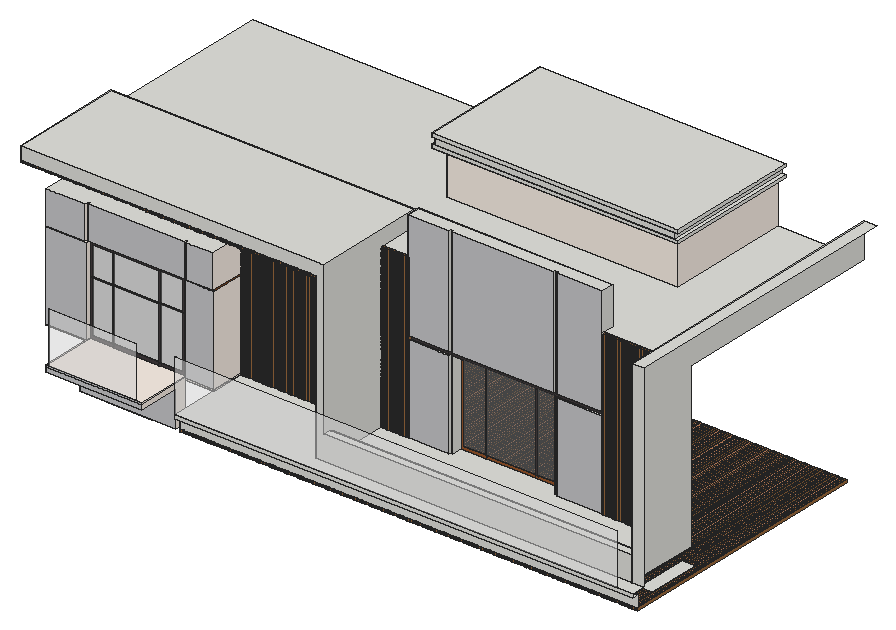
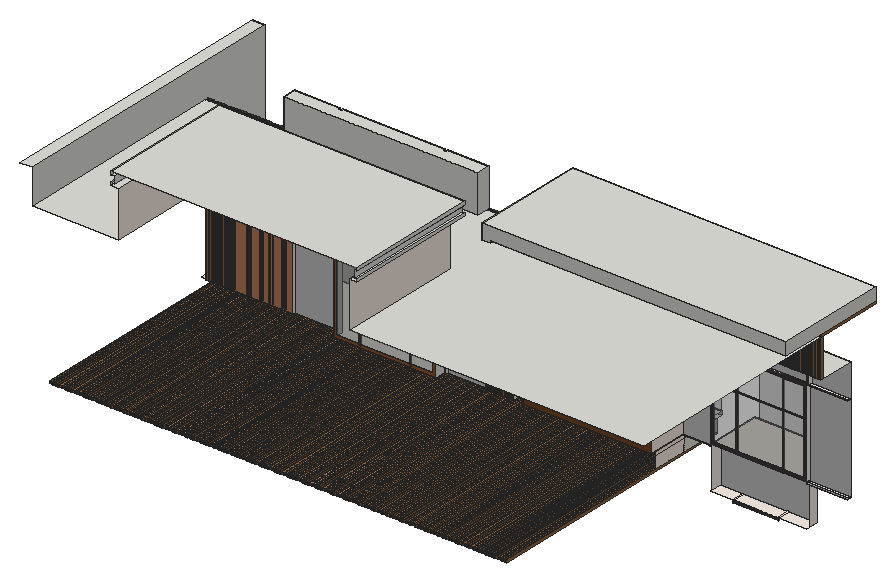
# SketchUp Ruby script. Lengths in inches.
U = 1.inch
M = Sketchup.active_model
def pt(a) = Geom::Point3d.new(a.map { |v| v * U })
def face(e, loops, mat)
  f = e.add_face(loops[0].map { |a| pt(a) })
  loops[1..].each { |l| e.add_face(l.map { |a| pt(a) }).erase! }
  f.material = f.back_material = mat if mat
  f
end
# faces: each face lists its corners as indices into pts; further lists are holes
def faces(e, pts, list, mat = nil) = list.each { |f| face(e, (f[0].is_a?(Array) ? f : [f]).map { |l| l.map { |i| pts[i] } }, mat) }
# xy, xz, yz: faces in a plane at the given z, y or x. An outline is a flat list of corners, or four numbers for a rectangle; further outlines are holes
def ring(l) = l.size == 4 ? [[l[0], l[1]], [l[2], l[1]], [l[2], l[3]], [l[0], l[3]]] : l.each_slice(2).to_a
def flat(e, list, mat, &to3) = list.each { |f| face(e, (f[0].is_a?(Array) ? f : [f]).map { |l| ring(l).map { |u, v| to3.(u, v) } }, mat) }
def xy(e, z, list, mat = nil) = flat(e, list, mat) { |x, y| [x, y, z] }
def xz(e, y, list, mat = nil) = flat(e, list, mat) { |x, z| [x, y, z] }
def yz(e, x, list, mat = nil) = flat(e, list, mat) { |y, z| [x, y, z] }
def lines(e, pts, list) = list.each { |a, b| e.add_line(pt(pts[a]), pt(pts[b])) }
# prism: a flat outline (further loops are holes) pulled along v
def prism(e, loops, v, mat = nil)
  f = face(e, loops, mat); d = Geom::Vector3d.new(v.map { |x| x * U })
  f.pushpull(f.normal.samedirection?(d) ? d.length : -d.length)
end
def box(e, o, s, mat = nil) = prism(e, [[o, [o[0] + s[0], o[1], o[2]], [o[0] + s[0], o[1] + s[1], o[2]], [o[0], o[1] + s[1], o[2]]]], [0, 0, s[2]], mat)
def at(x, y, z, deg = 0) = Geom::Transformation.translation(pt([x, y, z])) * Geom::Transformation.rotation(ORIGIN, Z_AXIS, deg.degrees)
def axes(o, x, y, z) = Geom::Transformation.new([*x, 0, *y, 0, *z, 0, *pt(o).to_a, 1])
def part(name) = M.definitions.add(name)
# library, detail: a bought-in or finely detailed component or shape, given as its bounding box
def library(name, o, s) = part(name).tap { |d| box(d.entities, o, s) }
def detail(e, o, s) = box(e.add_group.entities, o, s)
def put(e, d, t, mat = nil) = e.add_instance(d, t).tap { |i| i.material = mat if mat }
def group(e, t, mat = nil) = e.add_group.tap { |g| g.transformation = t; g.material = mat if mat }.entities
root = M.entities
M.materials.add("Resin FOG").color = [255, 255, 255]
M.materials["Resin FOG"].alpha = 0.29
M.materials.add("[0009_Linen]").color = [250, 240, 230]
M.materials.add("[Asphalt New]").color = [67, 60, 62]
M.materials.add("[Polished Concrete New]").color = [200, 200, 203]
M.materials.add("[Translucent Glass Gray]").color = [128, 128, 128]
M.materials["[Translucent Glass Gray]"].alpha = 0.5
M.materials.add("[Wood Cherry Original]").color = [152, 86, 42]
M.materials.add("[Wood Floor]").color = [155, 105, 61]
M.materials.add("[Wood Veneer 01]").color = [120, 70, 37]
M.materials.add("[Wood Veneer 02]").color = [190, 128, 91]
c1 = part("Group\#2")
xy(c1.entities,0,[[0,0,1.85,1.85],[2.64,0,4.49,1.85],[5.28,0,7.125,1.85],[7.91,0,9.76,1.85],[10.55,0,12.4,1.85],
  [13.1875,0,15.04,1.85],[15.83,0,17.68,1.85],[18.46,0,20.31,1.85],[21.1,0,22.95,1.85]],"[Wood Floor]")
g1 = group(c1.entities,at(0,0,0))
xy(g1,112.2,[[0,0,1.85,1.85],[2.64,0,4.49,1.85],[5.28,0,7.125,1.85],[7.91,0,9.76,1.85],[10.55,0,12.4,1.85],
  [13.1875,0,15.04,1.85],[15.83,0,17.68,1.85],[18.46,0,20.31,1.85],[21.1,0,22.95,1.85]],"[Wood Floor]")
xz(g1,0,[[0,0,1.85,112.2],[2.64,0,4.49,112.2],[5.28,0,7.125,112.2],[7.91,0,9.76,112.2],[10.55,0,12.4,112.2],
  [13.1875,0,15.04,112.2],[15.83,0,17.68,112.2],[18.46,0,20.31,112.2],[21.1,0,22.95,112.2]],"[Wood Floor]")
xz(g1,1.85,[[0,0,1.85,112.2],[2.64,0,4.49,112.2],[5.28,0,7.125,112.2],[7.91,0,9.76,112.2],[10.55,0,12.4,112.2],
  [13.1875,0,15.04,112.2],[15.83,0,17.68,112.2],[18.46,0,20.31,112.2],[21.1,0,22.95,112.2]],"[Wood Floor]")
yz(g1,0,[[0,0,1.85,112.2]],"[Wood Floor]")
yz(g1,1.85,[[0,0,1.85,112.2]],"[Wood Floor]")
yz(g1,2.64,[[0,0,1.85,112.2]],"[Wood Floor]")
yz(g1,4.49,[[0,0,1.85,112.2]],"[Wood Floor]")
yz(g1,5.28,[[0,0,1.85,112.2]],"[Wood Floor]")
yz(g1,7.125,[[0,0,1.85,112.2]],"[Wood Floor]")
yz(g1,7.91,[[0,0,1.85,112.2]],"[Wood Floor]")
yz(g1,9.76,[[0,0,1.85,112.2]],"[Wood Floor]")
yz(g1,10.55,[[0,0,1.85,112.2]],"[Wood Floor]")
yz(g1,12.4,[[0,0,1.85,112.2]],"[Wood Floor]")
yz(g1,13.1875,[[0,0,1.85,112.2]],"[Wood Floor]")
yz(g1,15.04,[[0,0,1.85,112.2]],"[Wood Floor]")
yz(g1,15.83,[[0,0,1.85,112.2]],"[Wood Floor]")
yz(g1,17.68,[[0,0,1.85,112.2]],"[Wood Floor]")
yz(g1,18.46,[[0,0,1.85,112.2]],"[Wood Floor]")
yz(g1,20.31,[[0,0,1.85,112.2]],"[Wood Floor]")
yz(g1,21.1,[[0,0,1.85,112.2]],"[Wood Floor]")
yz(g1,22.95,[[0,0,1.85,112.2]],"[Wood Floor]")
c2 = part("glass")
p = [[-167.89,-148.66,14.5],[-167.89,-148.66,14.51],[-167.89,-148.66,14.52]]
lines(c2.entities,p,[[0,1],[1,2]])
g2 = group(c2.entities,at(-34.63,-28.25,2))
box(g2,[0,0,0],[93.3125,0.375,32.75],"Resin FOG")
xy(root,216.73,[[160.07,282.18,208.29,304.24],[208.29,282.18,210.23,304.24],[210.23,282.18,286.57,304.24],[286.57,282.18,288.77,304.24],[288.77,282.18,328.15,304.24]],"[0009_Linen]")
xy(root,258.1,[[378.25,228.43,378.25,359.87,606.93,359.87,606.93,683.93,813.49,683.93,813.49,228.43],[813.49,228.43,1174.71,683.93]],"[Wood Veneer 02]")
xy(root,272.3125,[[1155.46,256.56,1176.625,349.72]])
xy(root,278.83,[[160.07,208.18,328.15,282.18]],"[Polished Concrete New]")
xy(root,278.88,[[378.25,216.68,1174.71,228.43]])
xy(root,285.125,[[378.25,216.68,1174.71,216.68,1174.71,242.24,602.83,242.24,602.83,369.43,378.25,369.43],[617.65,256.58,1153.77,256.58,1153.77,369.43,1002.71,369.43,1002.71,366.12,923.15,366.12,923.15,369.43,918.24,369.43,918.24,386.43,740.27,386.43,740.27,369.43,736.21,369.43,736.21,366.12,664.06,366.12,664.06,369.43,617.65,369.43]])
xy(root,285.125,[[328.15,300.43,378.25,301.37]],"[0009_Linen]")
xy(root,287.46,[[328.15,301.37,378.25,301.87]],"[0009_Linen]")
xy(root,287.46,[[88.9375,298.43,160.07,304.24]],"[Polished Concrete New]")
xy(root,289.58,[[160.07,208.18,328.15,304.24],[88.9375,298.43,160.07,304.24]],"[0009_Linen]")
xy(root,327.83,[[617.65,242.24,1153.77,256.58]])
xy(root,437.75,[[664.06,366.12,736.21,369.43],[923.15,366.12,1002.71,369.43],[740.27,369.43,918.24,386.43]])
xy(root,440.17,[[328.15,301.87,378.25,304.24]],"[0009_Linen]")
xy(root,440.86,[[88.9375,298.43,160.07,304.24]],"[0009_Linen]")
xy(root,442.55,[[88.9375,298.43,157.11,304.24],[160.07,300.43,328.15,304.24],[329.89,300.43,378.25,304.24]],"[0009_Linen]")
xy(root,444.14,[[664.06,366.12,736.21,369.43],[740.27,366.12,918.24,369.43],[923.15,366.12,1002.71,369.43]])
xy(root,500.25,[[88.9375,298.43,157.11,298.43,157.11,304.24,160.07,304.24,160.07,300.43,328.15,300.43,328.15,304.24,329.89,304.24,329.89,300.43,378.25,300.43,378.25,363.07,88.9375,363.07],[378.25,363.07,599.77,369.43]])
xy(root,566.3125,[[88.9375,363.07,599.77,363.07,599.77,369.43,602.83,369.43,602.83,439.5,617.65,439.5,617.65,369.43,664.06,369.43,664.06,389.3125,1002.71,389.3125,1002.71,369.43,1153.77,369.43,1153.77,747.375,1002.71,747.375,1002.71,529.6,601.41,529.6,601.41,747.375,88.9375,747.375]])
xy(root,570.3,[[88.9375,242.24,602.83,439.5]])
xy(root,591.9375,[[88.9375,242.24,617.65,439.5]])
xy(root,626.3125,[[1153.77,242.24,1174.71,747.375]])
xy(root,632.0625,[[664.06,366.12,736.21,366.12,736.21,369.43,740.27,369.43,740.27,366.12,918.24,366.12,918.24,369.43,923.15,369.43,923.15,366.12,1002.71,366.12,1002.71,389.3125,664.06,389.3125]])
xy(root,646.01,[[588.47,512.47,601.41,747.375],[601.41,512.47,1016.65,529.6],[1002.71,529.6,1016.65,747.375]])
xy(root,651.03,[[588.47,512.47,1009.71,515.03],[1009.71,512.47,1016.65,747.375],[588.47,515.03,592.41,747.375]])
xy(root,662.48,[[588.47,512.47,1016.65,515.03],[588.47,515.03,592.41,747.375],[1009.71,515.03,1016.65,747.375]])
xy(root,668.375,[[588.47,512.47,1016.65,747.375]])
xz(root,208.18,[[160.07,278.83,328.15,287.46],[160.07,287.46,328.15,289.58]],"[Polished Concrete New]")
xz(root,216.68,[[378.25,278.88,1174.71,285.125]])
xz(root,228.43,[[378.25,258.1,1174.71,278.88]])
xz(root,242.24,[[602.83,285.125,1153.77,285.125,1153.77,327.83,617.65,327.83,617.65,591.9375,88.9375,591.9375,88.9375,570.3,602.83,570.3],[1153.77,285.125,1174.71,626.3125]])
xz(root,256.58,[[617.65,285.125,1153.77,327.83]])
xz(root,282.18,[[160.07,216.73,328.15,278.83]],"[Polished Concrete New]")
xz(root,298.43,[[88.9375,289.58,160.07,440.86],[88.9375,442.55,157.11,500.25]],"[Polished Concrete New]")
xz(root,300.43,[[160.07,442.55,328.15,500.25],[329.89,442.55,378.25,500.25]],"[Polished Concrete New]")
xz(root,301.37,[[328.15,285.125,378.25,287.46]],"[0009_Linen]")
xz(root,301.87,[[328.15,287.46,378.25,440.17]],"[Polished Concrete New]")
xz(root,304.24,[[88.9375,287.46,160.07,289.58],[328.15,440.17,378.25,442.55],[88.9375,440.86,160.07,442.55],[157.11,442.55,160.07,500.25],[328.15,442.55,329.89,500.25]],"[0009_Linen]")
xz(root,304.24,[[208.29,212.5,210.23,216.73],[210.23,212.5,286.57,216.73],[286.57,212.5,288.77,216.73],[160.07,289.58,200.14,289.58,200.14,295,165.49,295,165.49,385.92,160.07,385.92],[200.14,289.58,201.67,295],
  [201.67,289.58,281,295],[281,289.58,283.3125,295],[283.3125,289.58,328.15,289.58,328.15,385.92,322.73,385.92,322.73,295,283.3125,295],[200.14,295,201.67,385.92],[281,295,283.3125,385.92],
  [160.07,385.92,165.49,387.39],[165.49,385.92,200.14,387.39],[200.14,385.92,201.67,387.39],[201.67,385.92,281,387.39],[281,385.92,283.3125,387.39],
  [283.3125,385.92,322.73,387.39],[322.73,385.92,328.15,387.39],[160.07,387.39,165.49,387.39,165.49,437.13,200.14,437.13,200.14,442.55,160.07,442.55],[200.14,387.39,201.67,437.13],[281,387.39,283.3125,437.13],
  [322.73,387.39,328.15,387.39,328.15,442.55,283.3125,442.55,283.3125,437.13,322.73,437.13],[200.14,437.13,201.67,442.55],[201.67,437.13,281,442.55],[281,437.13,283.3125,442.55]],"[Asphalt New]")
xz(root,304.24,[[165.49,295,200.14,385.92],[201.67,295,281,385.92],[283.3125,295,322.73,385.92],[165.49,387.39,200.14,437.13],[201.67,387.39,281,437.13],
  [283.3125,387.39,322.73,437.13]],"[Translucent Glass Gray]")
xz(root,363.07,[[88.9375,500.25,378.25,566.3125],[378.25,500.25,599.77,566.3125]],"[Wood Veneer 01]")
xz(root,366.12,[[664.06,285.125,736.21,437.75],[923.15,285.125,1002.71,437.75],[664.06,444.14,736.21,632.0625],[740.27,444.14,918.24,632.0625],[923.15,444.14,1002.71,632.0625]],"[Polished Concrete New]")
xz(root,369.43,[[736.21,285.125,740.27,437.75],[918.24,285.125,923.15,437.75],[664.06,437.75,736.21,444.14],[736.21,437.75,740.27,444.14],[740.27,437.75,918.24,444.14],
  [918.24,437.75,923.15,444.14],[923.15,437.75,1002.71,444.14],[736.21,444.14,740.27,632.0625],[918.24,444.14,923.15,632.0625]],"[Asphalt New]")
xz(root,369.43,[[378.25,285.125,602.83,285.125,602.83,566.3125,599.77,566.3125,599.77,500.25,378.25,500.25],[617.65,285.125,664.06,566.3125]],"[Wood Veneer 01]")
xz(root,369.43,[[1002.71,285.125,1153.77,566.3125]],"[Wood Veneer 02]")
xz(root,386.43,[[783.48,290.36,785.51,432.52],[871.28,290.36,874.06,432.52]],"[Asphalt New]")
xz(root,386.43,[[745.5,290.36,783.48,432.52],[785.51,290.36,871.28,432.52],[874.06,290.36,913,432.52]],"[Translucent Glass Gray]")
xz(root,386.43,[[740.27,285.125,783.48,285.125,783.48,290.36,745.5,290.36,745.5,432.52,871.28,432.52,871.28,437.75,740.27,437.75],[783.48,285.125,785.51,290.36],[785.51,285.125,871.28,290.36],[871.28,285.125,874.06,290.36],[874.06,285.125,918.24,285.125,918.24,437.75,874.06,437.75,874.06,432.52,913,432.52,913,290.36,874.06,290.36],
  [871.28,432.52,874.06,437.75]],"[Wood Cherry Original]")
xz(root,389.3125,[[664.06,566.3125,1002.71,632.0625]])
xz(root,439.5,[[602.83,566.3125,602.83,570.3,88.9375,570.3,88.9375,591.9375,617.65,591.9375,617.65,566.3125]])
xz(root,512.47,[[588.47,646.01,1016.65,651.03],[588.47,662.48,1016.65,668.375]])
xz(root,515.03,[[592.41,651.03,1009.71,662.48]])
xz(root,529.6,[[601.41,566.3125,1002.71,646.01]],"[0009_Linen]")
yz(root,88.9375,[[242.24,570.3,439.5,591.9375]])
yz(root,157.11,[[298.43,442.55,304.24,500.25]],"[0009_Linen]")
yz(root,160.07,[[282.18,216.73,282.18,278.83,208.18,278.83,208.18,287.46,298.43,287.46,298.43,216.73],[208.18,287.46,300.68,289.58],[300.68,287.46,304.24,289.58],[298.43,289.58,304.24,440.86],[300.43,442.55,304.24,500.25]],"[0009_Linen]")
yz(root,328.15,[[282.18,216.73,300.43,216.73,300.43,285.125,301.37,285.125,301.37,287.46,208.18,287.46,208.18,278.83,282.18,278.83],[208.18,287.46,301.87,289.58],[301.87,289.58,304.24,440.17],[300.43,442.55,304.24,500.25]],"[0009_Linen]")
yz(root,329.89,[[300.43,442.55,304.24,500.25]],"[0009_Linen]")
yz(root,378.25,[[228.43,258.1,300.43,278.88]])
yz(root,378.25,[[300.43,258.1,359.87,278.88],[300.43,278.88,359.87,285.125],[301.37,285.125,369.43,287.46],[301.87,287.46,369.43,440.17],[300.43,442.55,369.43,500.25]],"[0009_Linen]")
yz(root,378.25,[[304.24,440.17,369.43,442.55]],"[Wood Veneer 01]")
yz(root,588.47,[[512.47,646.01,747.375,651.03],[512.47,662.48,747.375,668.375]])
yz(root,592.41,[[515.03,651.03,747.375,662.48]])
yz(root,599.77,[[363.07,500.25,369.43,566.3125]])
yz(root,601.41,[[529.6,566.3125,747.375,646.01]],"[0009_Linen]")
yz(root,602.83,[[242.24,285.125,242.24,570.3,439.5,570.3,439.5,566.3125,369.43,566.3125,369.43,285.125]])
yz(root,617.65,[[256.58,285.125,369.43,285.125,369.43,566.3125,439.5,566.3125,439.5,591.9375,242.24,591.9375,242.24,327.83,256.58,327.83]])
yz(root,664.06,[[366.12,285.125,369.43,437.75],[366.12,444.14,369.43,566.3125],[366.12,566.3125,389.3125,632.0625]])
yz(root,736.21,[[366.12,285.125,369.43,437.75],[366.12,444.14,369.43,632.0625]])
yz(root,740.27,[[369.43,285.125,386.43,437.75],[366.12,444.14,369.43,632.0625]])
yz(root,918.24,[[369.43,285.125,386.43,437.75],[366.12,444.14,369.43,632.0625]])
yz(root,923.15,[[366.12,285.125,369.43,437.75],[366.12,444.14,369.43,632.0625]])
yz(root,1002.71,[[366.12,285.125,369.43,437.75],[366.12,444.14,369.43,566.3125],[366.12,566.3125,389.3125,632.0625]])
yz(root,1002.71,[[529.6,566.3125,747.375,646.01]],"[0009_Linen]")
yz(root,1009.71,[[515.03,651.03,747.375,662.48]])
yz(root,1016.65,[[512.47,646.01,747.375,651.03],[512.47,662.48,747.375,668.375]])
yz(root,1153.77,[[242.24,285.125,256.58,327.83],[256.58,285.125,256.58,327.83,242.24,327.83,242.24,626.3125,747.375,626.3125,747.375,566.3125,369.43,566.3125,369.43,285.125]])
p = [[599.77,363.07,500.25],[599.77,359.76,500.25],[664.06,365.51,457.03],[664.06,365.51,463.39]]
lines(root,p,[[0,1],[2,3]])
put(root,c1,axes([1125.875,228.43,258.1],[2.12,0,0],[0,0,-2.12],[0,4.05957,0]))
put(root,c1,axes([1077.8125,228.43,258.1],[2.12,0,0],[0,0,-2.12],[0,4.05957,0]))
put(root,c1,axes([1029.75,228.43,258.1],[2.12,0,0],[0,0,-2.12],[0,4.05957,0]))
put(root,c1,axes([981.6875,228.43,258.1],[2.12,0,0],[0,0,-2.12],[0,4.05957,0]))
put(root,c1,axes([933.625,228.43,258.1],[2.12,0,0],[0,0,-2.12],[0,4.05957,0]))
put(root,c1,axes([885.5625,228.43,258.1],[2.12,0,0],[0,0,-2.12],[0,4.05957,0]))
put(root,c1,axes([837.5,228.43,258.1],[2.12,0,0],[0,0,-2.12],[0,4.05957,0]))
put(root,c1,axes([788.5625,228.43,258.1],[2.12,0,0],[0,0,-2.12],[0,4.05957,0]))
put(root,c1,axes([739.625,228.43,258.1],[2.12,0,0],[0,0,-2.12],[0,4.05957,0]))
put(root,c1,axes([690.6875,228.43,258.1],[2.12,0,0],[0,0,-2.12],[0,4.05957,0]))
put(root,c1,axes([641.75,228.43,258.1],[2.12,0,0],[0,0,-2.12],[0,4.05957,0]))
put(root,c1,axes([592.8125,228.43,258.1],[2.12,0,0],[0,0,-2.12],[0,4.05957,0]))
put(root,c1,axes([543.875,228.43,258.1],[2.12,0,0],[0,0,-2.12],[0,4.05957,0]))
put(root,c1,axes([494.9375,228.43,258.1],[2.12,0,0],[0,0,-2.12],[0,4.05957,0]))
put(root,c1,axes([446.6875,228.43,258.1],[2.12,0,0],[0,0,-2.12],[0,4.05957,0]))
put(root,c1,axes([399.4375,228.43,258.1],[2.12,0,0],[0,0,-2.12],[0,4.05957,0]))
put(root,c1,axes([378.25,228.43,258.1],[2.12,0,0],[0,0,-2.12],[0,4.05957,0]))
put(root,c1,axes([560.625,359.76,285.125],[2.12,0,0],[0,2.12,0],[0,0,2.52004]))
put(root,c1,axes([511.0625,359.76,285.125],[2.12,0,0],[0,2.12,0],[0,0,2.52004]))
put(root,c2,axes([664.1,244.93,279.64],[8.25497,0,0],[0,1,0],[0,0,2.74]))
put(root,c1,axes([1105.11,365.51,285.125],[2.12,0,0],[0,2.12,0],[0,0,2.50602]))
put(root,c1,axes([1055.41,364.24,285.125],[2.12,0,0],[0,2.12,0],[0,0,2.50602]))
put(root,c1,axes([1005.91,364.24,285.125],[2.12,0,0],[0,2.12,0],[0,0,2.50602]))
put(root,c1,axes([617.65,365.51,285.125],[2.12,0,0],[0,2.12,0],[0,0,2.50602]))
put(root,c1,axes([378.25,359.87,285.125],[2.12,0,0],[0,2.12,0],[0,0,2.52004]))
put(root,c1,axes([462.625,359.76,285.125],[2.12,0,0],[0,2.12,0],[0,0,2.52004]))
put(root,c1,axes([416.625,359.76,285.125],[2.12,0,0],[0,2.12,0],[0,0,2.52004]))
put(root,c2,axes([223.5625,236.06,284.1],[1.63713,0,0],[0,1,0],[0,0,2.74]))
put(root,c1,axes([327.98,359.15,500.25],[2.12,0,0],[0,2.12,0],[0,0,0.58877]))
put(root,c1,axes([279.32,359.15,500.25],[2.12,0,0],[0,2.12,0],[0,0,0.58877]))
put(root,c1,axes([231.94,359.15,500.25],[2.12,0,0],[0,2.12,0],[0,0,0.58877]))
put(root,c1,axes([183.28,359.15,500.25],[2.12,0,0],[0,2.12,0],[0,0,0.58877]))
put(root,c1,axes([134.625,359.15,500.25],[2.12,0,0],[0,2.12,0],[0,0,0.58877]))
put(root,c1,axes([88.9375,359.15,500.25],[2.12,0,0],[0,2.12,0],[0,0,0.58877]))
put(root,c1,axes([409.42,242.24,570.3],[2.12,0,0],[0,0,-2.12],[0,1.04732,0]))
put(root,c1,axes([358.86,242.24,570.3],[2.12,0,0],[0,0,-2.12],[0,1.04732,0]))
put(root,c1,axes([307.98,242.24,570.3],[2.12,0,0],[0,0,-2.12],[0,1.04732,0]))
put(root,c1,axes([262.55,243.73,570.3],[2.12,0,0],[0,0,-2.12],[0,1.04732,0]))
put(root,c1,axes([213.48,243.73,570.3],[2.12,0,0],[0,0,-2.12],[0,1.04732,0]))
put(root,c1,axes([164.42,243.73,570.3],[2.12,0,0],[0,0,-2.12],[0,1.04732,0]))
put(root,c1,axes([115.36,243.73,570.3],[2.12,0,0],[0,0,-2.12],[0,1.04732,0]))
put(root,c1,axes([88.9375,243.73,570.3],[1.13352,0,0],[0,0,-2.12],[0,1.04732,0]))
put(root,c1,axes([554.17,242.24,570.3],[2.12,0,0],[0,0,-2.12],[0,1.04732,0]))
put(root,c1,axes([505.92,242.24,570.3],[2.12,0,0],[0,0,-2.12],[0,1.04732,0]))
put(root,c1,axes([456.67,242.24,570.3],[2.12,0,0],[0,0,-2.12],[0,1.04732,0]))
